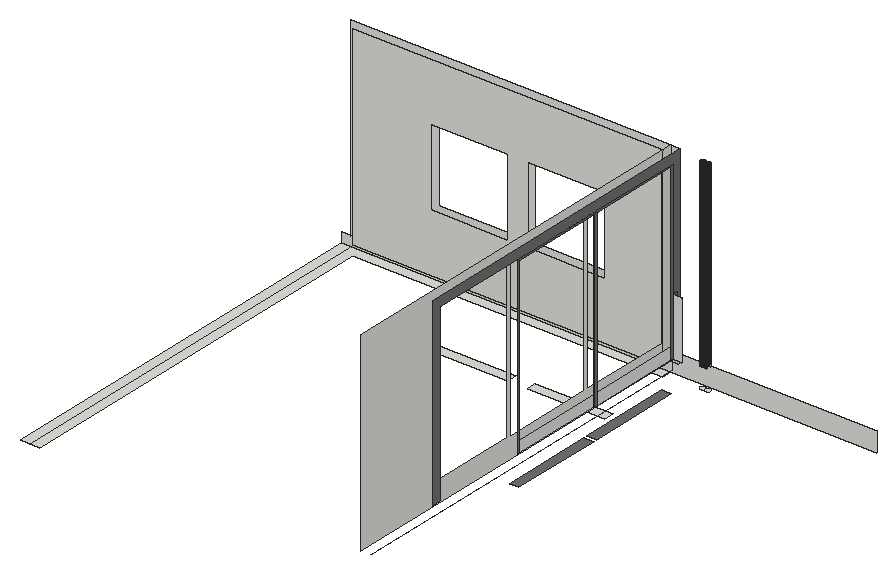
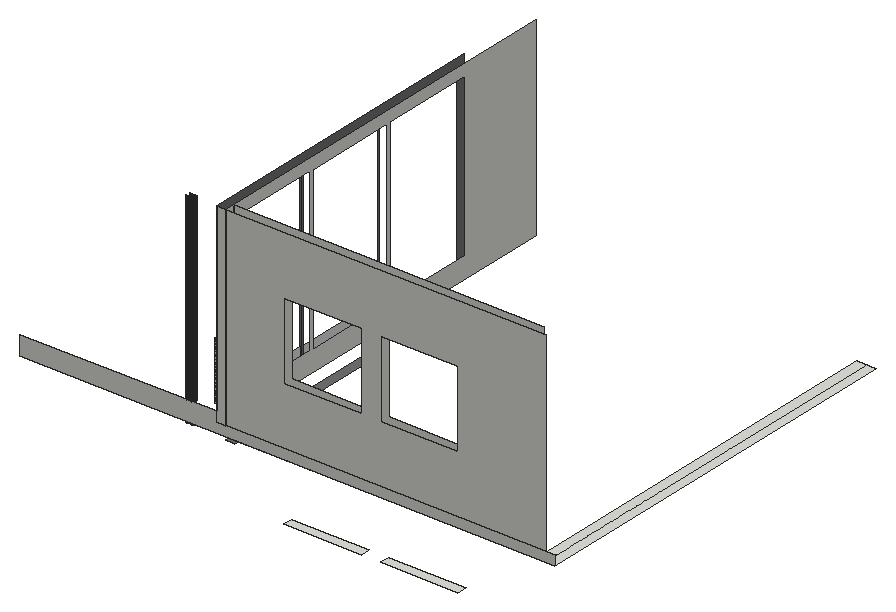
# SketchUp Ruby script. Lengths in inches.
U = 1.inch
M = Sketchup.active_model
def pt(a) = Geom::Point3d.new(a.map { |v| v * U })
def face(e, loops, mat)
  f = e.add_face(loops[0].map { |a| pt(a) })
  loops[1..].each { |l| e.add_face(l.map { |a| pt(a) }).erase! }
  f.material = f.back_material = mat if mat
  f
end
# faces: each face lists its corners as indices into pts; further lists are holes
def faces(e, pts, list, mat = nil) = list.each { |f| face(e, (f[0].is_a?(Array) ? f : [f]).map { |l| l.map { |i| pts[i] } }, mat) }
# xy, xz, yz: faces in a plane at the given z, y or x. An outline is a flat list of corners, or four numbers for a rectangle; further outlines are holes
def ring(l) = l.size == 4 ? [[l[0], l[1]], [l[2], l[1]], [l[2], l[3]], [l[0], l[3]]] : l.each_slice(2).to_a
def flat(e, list, mat, &to3) = list.each { |f| face(e, (f[0].is_a?(Array) ? f : [f]).map { |l| ring(l).map { |u, v| to3.(u, v) } }, mat) }
def xy(e, z, list, mat = nil) = flat(e, list, mat) { |x, y| [x, y, z] }
def xz(e, y, list, mat = nil) = flat(e, list, mat) { |x, z| [x, y, z] }
def yz(e, x, list, mat = nil) = flat(e, list, mat) { |y, z| [x, y, z] }
def lines(e, pts, list) = list.each { |a, b| e.add_line(pt(pts[a]), pt(pts[b])) }
# prism: a flat outline (further loops are holes) pulled along v
def prism(e, loops, v, mat = nil)
  f = face(e, loops, mat); d = Geom::Vector3d.new(v.map { |x| x * U })
  f.pushpull(f.normal.samedirection?(d) ? d.length : -d.length)
end
def box(e, o, s, mat = nil) = prism(e, [[o, [o[0] + s[0], o[1], o[2]], [o[0] + s[0], o[1] + s[1], o[2]], [o[0], o[1] + s[1], o[2]]]], [0, 0, s[2]], mat)
def at(x, y, z, deg = 0) = Geom::Transformation.translation(pt([x, y, z])) * Geom::Transformation.rotation(ORIGIN, Z_AXIS, deg.degrees)
def axes(o, x, y, z) = Geom::Transformation.new([*x, 0, *y, 0, *z, 0, *pt(o).to_a, 1])
def part(name) = M.definitions.add(name)
# library, detail: a bought-in or finely detailed component or shape, given as its bounding box
def library(name, o, s) = part(name).tap { |d| box(d.entities, o, s) }
def detail(e, o, s) = box(e.add_group.entities, o, s)
def put(e, d, t, mat = nil) = e.add_instance(d, t).tap { |i| i.material = mat if mat }
def group(e, t, mat = nil) = e.add_group.tap { |g| g.transformation = t; g.material = mat if mat }.entities
root = M.entities
M.materials.add("M01_Silver_Fog").color = [224, 224, 224]
M.materials.add("M06_Steel_Smoke").color = [114, 114, 114]
xy(root,474,[[60,474,108,480],[120,474,168,480]])
xy(root,503,[[204,355,210,413],[204,415,210,473]],"M06_Steel_Smoke")
xy(root,509.24,[[225.03,477.03,225.29,477.03,225.38,477.04,225.46,477.06,225.55,477.08,225.71,477.14,225.87,477.22,225.95,477.27,226.02,477.32,226.08,477.38,226.15,477.4375,226.21,477.5,226.26,477.57,226.32,477.64,226.36,477.72,226.4,477.79,226.44,477.875,226.47,477.96,226.5,478.04,226.54,478.21,226.55,478.3,226.55,478.5625,226.54,478.65,226.52,478.74,226.5,478.82,226.47,478.9,226.4375,478.99,226.4,479.07,226.36,479.14,226.3125,479.22,226.26,479.29,226.2,479.35,226.14,479.42,226.08,479.48,226.01,479.53,225.9375,479.59,225.86,479.63,225.79,479.68,225.71,479.71,225.54,479.77,225.46,479.79,225.37,479.81,225.19,479.83,225.11,479.82,225.02,479.82,224.93,479.81,224.85,479.79,224.76,479.77,224.6,479.71,224.52,479.67,224.4375,479.63,224.36,479.58,224.29,479.53,224.23,479.47,224.16,479.41,224.1,479.35,224.05,479.28,223.99,479.21,223.95,479.13,223.91,479.06,223.87,478.98,223.84,478.9,223.81,478.8125,223.79,478.73,223.77,478.64,223.76,478.55,223.76,478.29,223.77,478.2,223.8125,478.03,223.84,477.95,223.87,477.87,223.95,477.71,224,477.64,224.05,477.56,224.11,477.5,224.17,477.43,224.23,477.37,224.37,477.27,224.45,477.22,224.52,477.18,224.6,477.14,224.68,477.11,224.77,477.08,224.85,477.06,224.94,477.04],[228.34,477.03,228.6,477.03,228.69,477.04,228.78,477.06,228.86,477.08,228.95,477.11,229.03,477.14,229.11,477.18,229.18,477.22,229.26,477.27,229.33,477.32,229.4,477.38,229.46,477.4375,229.52,477.5,229.58,477.57,229.63,477.64,229.67,477.72,229.72,477.79,229.75,477.875,229.79,477.96,229.8125,478.04,229.83,478.125,229.85,478.21,229.87,478.39,229.87,478.47,229.86,478.5625,229.85,478.65,229.83,478.74,229.81,478.82,229.78,478.9,229.75,478.99,229.71,479.07,229.67,479.14,229.62,479.22,229.57,479.29,229.51,479.35,229.45,479.42,229.39,479.48,229.32,479.53,229.25,479.59,229.18,479.63,229.1,479.68,229.02,479.71,228.9375,479.74,228.85,479.77,228.77,479.79,228.68,479.81,228.59,479.82,228.51,479.83,228.42,479.82,228.33,479.82,228.24,479.81,228.16,479.79,228.07,479.77,227.91,479.71,227.75,479.63,227.61,479.53,227.47,479.41,227.41,479.35,227.31,479.21,227.26,479.13,227.22,479.06,227.18,478.98,227.15,478.9,227.12,478.8125,227.1,478.73,227.08,478.64,227.07,478.55,227.07,478.29,227.09,478.2,227.1,478.12,227.125,478.03,227.15,477.95,227.18,477.87,227.26,477.71,227.3125,477.64,227.36,477.56,227.42,477.5,227.48,477.43,227.54,477.37,227.68,477.27,227.76,477.22,227.84,477.18,227.91,477.14,228,477.11,228.08,477.08,228.17,477.06,228.25,477.04]],"M01_Silver_Fog")
xy(root,510,[[0,231,6,480],[6,231,6,480,204,480,204,474,12,474,12,231]])
xz(root,474,[[[12,516,204,636],[120,552,168,600],[60,552,108,600]]])
xz(root,474,[[210,522,215.53,558],[215.53,522,216,558]],"M01_Silver_Fog")
xz(root,477.03,[[225.03,522,225.12,635.24],[225.12,522,225.2,635.24],[225.2,522,225.29,635.24],[228.34,522,228.43,635.24],[228.43,522,228.52,635.24],
  [228.52,522,228.6,635.24]],"M01_Silver_Fog")
xz(root,479.82,[[225.02,522,225.11,635.24],[228.33,522,228.42,635.24]],"M01_Silver_Fog")
xz(root,480,[[0,510,0,516,210,516,210,522,331.55,522,331.55,510],[[6,516,204,636],[60,552,108,600],[120,552,168,600]],[204,516,210,636]])
yz(root,204,[[[240,516,474,636],[415,529,473,629],[295,529,353,629],[355,529,413,629]],[474,516,480,636]])
yz(root,210,[[355,522,413,529],[415,522,473,529]],"M01_Silver_Fog")
yz(root,210,[[288,522,294,522,294,630,474,630,474,558,477,558,477,522,480,522,480,636,288,636],[354,522,355,522,355,629,413,629,413,522,414,522,414,630,354,630],[414,522,415,522,415,629,473,629,473,522,474,522,474,630,414,630],[474,522,477,558]],"M06_Steel_Smoke")
yz(root,223.76,[[478.29,522,478.38,635.24],[478.38,522,478.47,635.24],[478.47,522,478.55,635.24]],"M01_Silver_Fog")
yz(root,226.55,[[478.3,522,478.39,635.24],[478.39,522,478.47,635.24],[478.47,522,478.5625,635.24]],"M01_Silver_Fog")
yz(root,227.07,[[478.29,522,478.38,635.24],[478.38,522,478.47,635.24],[478.47,522,478.55,635.24]],"M01_Silver_Fog")
p = [[224.85,477.06,522],[224.94,477.04,522],[224.94,477.04,635.24],[224.85,477.06,635.24],[225.03,477.03,522],[225.03,477.03,635.24],
  [225.29,477.03,522],[225.38,477.04,522],[225.38,477.04,635.24],[225.29,477.03,635.24],[225.46,477.06,522],[225.46,477.06,635.24],
  [228.17,477.06,522],[228.25,477.04,522],[228.25,477.04,635.24],[228.17,477.06,635.24],[228.34,477.03,522],[228.34,477.03,635.24],
  [228.6,477.03,522],[228.69,477.04,522],[228.69,477.04,635.24],[228.6,477.03,635.24],[228.78,477.06,522],[228.78,477.06,635.24],
  [224.52,477.18,522],[224.6,477.14,522],[224.6,477.14,635.24],[224.52,477.18,635.24],[224.68,477.11,522],[224.68,477.11,635.24],
  [224.77,477.08,522],[224.77,477.08,635.24],[225.55,477.08,522],[225.55,477.08,635.24],[225.63,477.11,522],[225.63,477.11,635.24],
  [225.71,477.14,522],[225.71,477.14,635.24],[225.79,477.18,522],[225.79,477.18,635.24],[227.84,477.18,522],[227.91,477.14,522],
  [227.91,477.14,635.24],[227.84,477.18,635.24],[228,477.11,522],[228,477.11,635.24],[228.08,477.08,522],[228.08,477.08,635.24],
  [228.86,477.08,522],[228.86,477.08,635.24],[228.95,477.11,522],[228.95,477.11,635.24],[229.03,477.14,522],[229.03,477.14,635.24],
  [224.37,477.27,522],[224.45,477.22,522],[224.45,477.22,635.24],[224.37,477.27,635.24],[225.87,477.22,522],[225.87,477.22,635.24],
  [225.95,477.27,522],[225.95,477.27,635.24],[227.68,477.27,522],[227.76,477.22,522],[227.76,477.22,635.24],[227.68,477.27,635.24],
  [224.23,477.37,522],[224.3,477.32,522],[224.3,477.32,635.24],[224.23,477.37,635.24],[226.02,477.32,522],[226.02,477.32,635.24],
  [226.08,477.38,522],[226.08,477.38,635.24],[227.54,477.37,522],[227.61,477.32,522],[227.61,477.32,635.24],[227.54,477.37,635.24],
  [224.11,477.5,522],[224.17,477.43,522],[224.17,477.43,635.24],[224.11,477.5,635.24],[226.15,477.4375,522],[226.15,477.4375,635.24],
  [226.21,477.5,522],[226.21,477.5,635.24],[227.42,477.5,522],[227.48,477.43,522],[227.48,477.43,635.24],[227.42,477.5,635.24],
  [224.05,477.56,522],[224.05,477.56,635.24],[226.26,477.57,522],[226.26,477.57,635.24],[227.36,477.56,522],[227.36,477.56,635.24],
  [223.95,477.71,522],[224,477.64,522],[224,477.64,635.24],[223.95,477.71,635.24],[226.32,477.64,522],[226.32,477.64,635.24],
  [226.36,477.72,522],[226.36,477.72,635.24],[227.26,477.71,522],[227.3125,477.64,522],[227.3125,477.64,635.24],[227.26,477.71,635.24],
  [223.91,477.79,522],[223.91,477.79,635.24],[226.4,477.79,522],[226.4,477.79,635.24],[227.22,477.79,522],[227.22,477.79,635.24],
  [223.87,477.87,522],[223.87,477.87,635.24],[226.44,477.875,522],[226.44,477.875,635.24],[227.18,477.87,522],[227.18,477.87,635.24],
  [223.8125,478.03,522],[223.84,477.95,522],[223.84,477.95,635.24],[223.8125,478.03,635.24],[226.47,477.96,522],[226.47,477.96,635.24],
  [227.125,478.03,522],[227.15,477.95,522],[227.15,477.95,635.24],[227.125,478.03,635.24],[223.79,478.12,522],[223.79,478.12,635.24],
  [226.5,478.04,522],[226.5,478.04,635.24],[226.52,478.125,522],[226.52,478.125,635.24],[227.1,478.12,522],[227.1,478.12,635.24],
  [223.77,478.2,522],[223.77,478.2,635.24],[226.54,478.21,522],[226.54,478.21,635.24],[227.09,478.2,522],[227.09,478.2,635.24],
  [223.76,478.29,522],[223.76,478.29,635.24],[226.55,478.3,522],[226.55,478.3,635.24],[227.07,478.29,522],[227.07,478.29,635.24],
  [223.77,478.64,522],[223.76,478.55,522],[223.76,478.55,635.24],[223.77,478.64,635.24],[223.79,478.73,522],[223.79,478.73,635.24],
  [226.54,478.65,522],[226.52,478.74,522],[226.52,478.74,635.24],[226.54,478.65,635.24],[226.55,478.5625,522],[226.55,478.5625,635.24],
  [227.08,478.64,522],[227.07,478.55,522],[227.07,478.55,635.24],[227.08,478.64,635.24],[227.1,478.73,522],[227.1,478.73,635.24],
  [223.81,478.8125,522],[223.81,478.8125,635.24],[226.5,478.82,522],[226.5,478.82,635.24],[227.12,478.8125,522],[227.12,478.8125,635.24],
  [223.84,478.9,522],[223.84,478.9,635.24],[226.47,478.9,522],[226.47,478.9,635.24],[227.15,478.9,522],[227.15,478.9,635.24],
  [223.87,478.98,522],[223.87,478.98,635.24],[226.4375,478.99,522],[226.4375,478.99,635.24],[227.18,478.98,522],[227.18,478.98,635.24],
  [223.91,479.06,522],[223.91,479.06,635.24],[226.4,479.07,522],[226.4,479.07,635.24],[227.22,479.06,522],[227.22,479.06,635.24],
  [223.95,479.13,522],[223.95,479.13,635.24],[223.99,479.21,522],[223.99,479.21,635.24],[226.36,479.14,522],[226.3125,479.22,522],
  [226.3125,479.22,635.24],[226.36,479.14,635.24],[227.26,479.13,522],[227.26,479.13,635.24],[227.31,479.21,522],[227.31,479.21,635.24],
  [224.05,479.28,522],[224.05,479.28,635.24],[226.26,479.29,522],[226.26,479.29,635.24],[227.36,479.28,522],[227.36,479.28,635.24],
  [224.1,479.35,522],[224.1,479.35,635.24],[224.16,479.41,522],[224.16,479.41,635.24],[226.2,479.35,522],[226.2,479.35,635.24],
  [227.41,479.35,522],[227.41,479.35,635.24],[227.47,479.41,522],[227.47,479.41,635.24],[224.23,479.47,522],[224.23,479.47,635.24],
  [226.14,479.42,522],[226.08,479.48,522],[226.08,479.48,635.24],[226.14,479.42,635.24],[227.54,479.47,522],[227.54,479.47,635.24],
  [224.29,479.53,522],[224.29,479.53,635.24],[224.36,479.58,522],[224.36,479.58,635.24],[226.01,479.53,522],[225.9375,479.59,522],
  [225.9375,479.59,635.24],[226.01,479.53,635.24],[227.61,479.53,522],[227.61,479.53,635.24],[227.68,479.58,522],[227.68,479.58,635.24],
  [224.4375,479.63,522],[224.4375,479.63,635.24],[224.52,479.67,522],[224.52,479.67,635.24],[225.86,479.63,522],[225.79,479.68,522],
  [225.79,479.68,635.24],[225.86,479.63,635.24],[227.75,479.63,522],[227.75,479.63,635.24],[227.83,479.67,522],[227.83,479.67,635.24],
  [224.6,479.71,522],[224.6,479.71,635.24],[224.68,479.74,522],[224.68,479.74,635.24],[224.76,479.77,522],[224.76,479.77,635.24],
  [225.625,479.74,522],[225.54,479.77,522],[225.54,479.77,635.24],[225.625,479.74,635.24],[225.71,479.71,522],[225.71,479.71,635.24],
  [227.91,479.71,522],[227.91,479.71,635.24],[227.99,479.74,522],[227.99,479.74,635.24],[228.07,479.77,522],[228.07,479.77,635.24],
  [228.9375,479.74,522],[228.85,479.77,522],[228.85,479.77,635.24],[228.9375,479.74,635.24],[229.02,479.71,522],[229.02,479.71,635.24],
  [224.85,479.79,522],[224.85,479.79,635.24],[224.93,479.81,522],[224.93,479.81,635.24],[225.02,479.82,522],[225.02,479.82,635.24],
  [225.19,479.83,522],[225.11,479.82,522],[225.11,479.82,635.24],[225.19,479.83,635.24],[225.28,479.82,522],[225.28,479.82,635.24],
  [225.37,479.81,522],[225.37,479.81,635.24],[225.46,479.79,522],[225.46,479.79,635.24],[228.16,479.79,522],[228.16,479.79,635.24],
  [228.24,479.81,522],[228.24,479.81,635.24],[228.33,479.82,522],[228.33,479.82,635.24],[228.51,479.83,522],[228.42,479.82,522],
  [228.42,479.82,635.24],[228.51,479.83,635.24],[228.59,479.82,522],[228.59,479.82,635.24],[228.68,479.81,522],[228.68,479.81,635.24],
  [228.77,479.79,522],[228.77,479.79,635.24],[210,240,516],[210,474,516],[210,474,522]]
faces(root,p,[[0,1,2,3],[1,4,5,2],[6,7,8,9],[7,10,11,8],[12,13,14,15],[13,16,17,14],[18,19,20,21],[19,22,23,20],
  [24,25,26,27],[25,28,29,26],[28,30,31,29],[30,0,3,31],[10,32,33,11],[32,34,35,33],[34,36,37,35],[36,38,39,37],
  [40,41,42,43],[41,44,45,42],[44,46,47,45],[46,12,15,47],[22,48,49,23],[48,50,51,49],[50,52,53,51],[54,55,56,57],
  [55,24,27,56],[38,58,59,39],[58,60,61,59],[62,63,64,65],[63,40,43,64],[66,67,68,69],[67,54,57,68],[60,70,71,61],
  [70,72,73,71],[74,75,76,77],[75,62,65,76],[78,79,80,81],[79,66,69,80],[72,82,83,73],[82,84,85,83],[86,87,88,89],
  [87,74,77,88],[90,78,81,91],[84,92,93,85],[94,86,89,95],[96,97,98,99],[97,90,91,98],[92,100,101,93],[100,102,103,101],
  [104,105,106,107],[105,94,95,106],[108,96,99,109],[102,110,111,103],[112,104,107,113],[114,108,109,115],[110,116,117,111],[118,112,113,119],
  [120,121,122,123],[121,114,115,122],[116,124,125,117],[126,127,128,129],[127,118,119,128],[130,120,123,131],[124,132,133,125],[132,134,135,133],
  [136,126,129,137],[138,130,131,139],[134,140,141,135],[142,136,137,143],[144,138,139,145],[140,146,147,141],[148,142,143,149],[150,151,152,153],
  [154,150,153,155],[156,157,158,159],[160,156,159,161],[162,163,164,165],[166,162,165,167],[168,154,155,169],[157,170,171,158],[172,166,167,173],
  [174,168,169,175],[170,176,177,171],[178,172,173,179],[180,174,175,181],[176,182,183,177],[184,178,179,185],[186,180,181,187],[182,188,189,183],
  [190,184,185,191],[192,186,187,193],[194,192,193,195],[196,197,198,199],[188,196,199,189],[200,190,191,201],[202,200,201,203],[204,194,195,205],
  [197,206,207,198],[208,202,203,209],[210,204,205,211],[212,210,211,213],[206,214,215,207],[216,208,209,217],[218,216,217,219],[220,212,213,221],
  [222,223,224,225],[214,222,225,215],[226,218,219,227],[228,220,221,229],[230,228,229,231],[232,233,234,235],[223,232,235,224],[236,226,227,237],
  [238,236,237,239],[240,230,231,241],[242,240,241,243],[244,245,246,247],[233,244,247,234],[248,238,239,249],[250,248,249,251],[252,242,243,253],
  [254,252,253,255],[256,254,255,257],[258,259,260,261],[262,258,261,263],[245,262,263,246],[264,250,251,265],[266,264,265,267],[268,266,267,269],
  [270,271,272,273],[274,270,273,275],[276,256,257,277],[278,276,277,279],[280,278,279,281],[282,283,284,285],[286,282,285,287],[288,286,287,289],
  [290,288,289,291],[259,290,291,260],[292,268,269,293],[294,292,293,295],[296,294,295,297],[298,299,300,301],[302,298,301,303],[304,302,303,305],
  [306,304,305,307],[271,306,307,272]],"M01_Silver_Fog")
lines(root,p,[[308,309],[309,310]])
